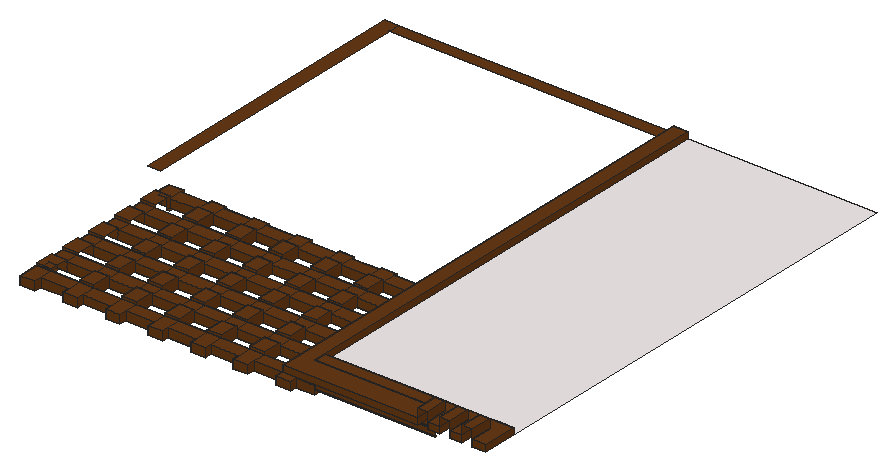
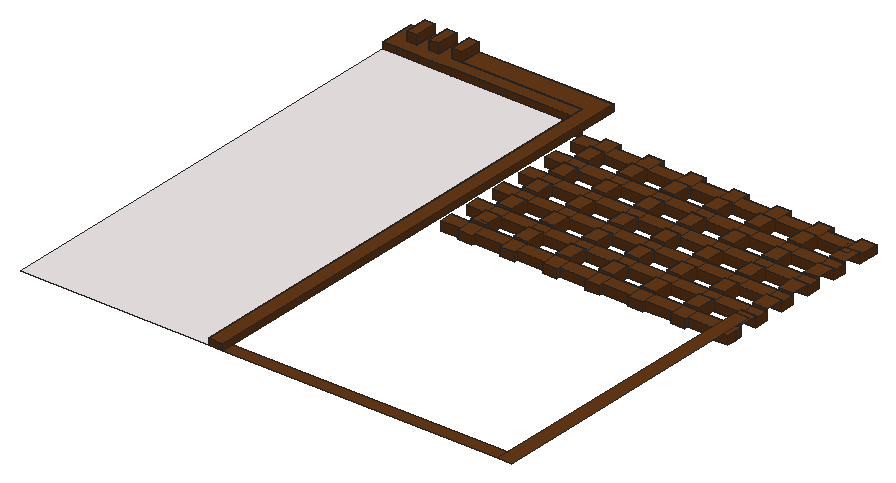
# SketchUp Ruby script. Lengths in inches.
U = 1.inch
M = Sketchup.active_model
def pt(a) = Geom::Point3d.new(a.map { |v| v * U })
def face(e, loops, mat)
  f = e.add_face(loops[0].map { |a| pt(a) })
  loops[1..].each { |l| e.add_face(l.map { |a| pt(a) }).erase! }
  f.material = f.back_material = mat if mat
  f
end
# faces: each face lists its corners as indices into pts; further lists are holes
def faces(e, pts, list, mat = nil) = list.each { |f| face(e, (f[0].is_a?(Array) ? f : [f]).map { |l| l.map { |i| pts[i] } }, mat) }
# xy, xz, yz: faces in a plane at the given z, y or x. An outline is a flat list of corners, or four numbers for a rectangle; further outlines are holes
def ring(l) = l.size == 4 ? [[l[0], l[1]], [l[2], l[1]], [l[2], l[3]], [l[0], l[3]]] : l.each_slice(2).to_a
def flat(e, list, mat, &to3) = list.each { |f| face(e, (f[0].is_a?(Array) ? f : [f]).map { |l| ring(l).map { |u, v| to3.(u, v) } }, mat) }
def xy(e, z, list, mat = nil) = flat(e, list, mat) { |x, y| [x, y, z] }
def xz(e, y, list, mat = nil) = flat(e, list, mat) { |x, z| [x, y, z] }
def yz(e, x, list, mat = nil) = flat(e, list, mat) { |y, z| [x, y, z] }
def lines(e, pts, list) = list.each { |a, b| e.add_line(pt(pts[a]), pt(pts[b])) }
# prism: a flat outline (further loops are holes) pulled along v
def prism(e, loops, v, mat = nil)
  f = face(e, loops, mat); d = Geom::Vector3d.new(v.map { |x| x * U })
  f.pushpull(f.normal.samedirection?(d) ? d.length : -d.length)
end
def box(e, o, s, mat = nil) = prism(e, [[o, [o[0] + s[0], o[1], o[2]], [o[0] + s[0], o[1] + s[1], o[2]], [o[0], o[1] + s[1], o[2]]]], [0, 0, s[2]], mat)
def at(x, y, z, deg = 0) = Geom::Transformation.translation(pt([x, y, z])) * Geom::Transformation.rotation(ORIGIN, Z_AXIS, deg.degrees)
def axes(o, x, y, z) = Geom::Transformation.new([*x, 0, *y, 0, *z, 0, *pt(o).to_a, 1])
def part(name) = M.definitions.add(name)
# library, detail: a bought-in or finely detailed component or shape, given as its bounding box
def library(name, o, s) = part(name).tap { |d| box(d.entities, o, s) }
def detail(e, o, s) = box(e.add_group.entities, o, s)
def put(e, d, t, mat = nil) = e.add_instance(d, t).tap { |i| i.material = mat if mat }
def group(e, t, mat = nil) = e.add_group.tap { |g| g.transformation = t; g.material = mat if mat }.entities
root = M.entities
M.materials.add("Generic").color = [102, 57, 22]
M.materials.add("Generic\#3").color = [243, 235, 235]
xy(root,493.22,[[27.12,205.01,30.01,205.01,30.01,218.57,19.57,218.57,19.57,208.75,27.12,208.75]],"Generic")
xy(root,493.4375,[[13.1875,47.8125,13.1875,67.5625,288.56,67.5625,288.56,54.375,270.5,54.375,270.5,47.8125,256.5625,47.8125,256.5625,54.375,229.93,54.375,229.93,47.8125,216,47.8125,216,54.375,189.37,54.375,189.37,47.8125,175.4375,47.8125,175.4375,54.375,148.81,54.375,148.81,47.8125,134.875,47.8125,134.875,54.375,108.25,54.375,108.25,47.8125,94.3125,47.8125,94.3125,54.375,67.68,54.375,67.68,47.8125,53.75,47.8125,53.75,54.375,27.12,54.375,27.12,47.8125],[53.75,67.5625,67.68,85.25],[94.3125,67.5625,108.25,85.25],[134.875,67.5625,148.81,85.25],[175.4375,67.5625,189.37,85.25],
  [216,67.5625,229.93,85.25],[256.5625,67.5625,270.5,85.25],[13.1875,85.25,288.56,98.4375],[53.75,98.4375,67.68,116.125],[94.3125,98.4375,108.25,116.125],
  [134.875,98.4375,148.81,116.125],[175.4375,98.4375,189.37,116.125],[216,98.4375,229.93,116.125],[256.5625,98.4375,270.5,116.125],[13.1875,116.125,288.56,129.3125],
  [53.75,129.3125,67.68,147],[94.3125,129.3125,108.25,147],[134.875,129.3125,148.81,147],[175.4375,129.3125,189.37,147],[216,129.3125,229.93,147],
  [256.5625,129.3125,270.5,147],[13.1875,147,288.56,160.1875],[53.75,160.1875,67.68,177.875],[94.3125,160.1875,108.25,177.875],[134.875,160.1875,148.81,177.875],
  [175.4375,160.1875,189.37,177.875],[216,160.1875,229.93,177.875],[256.5625,160.1875,270.5,177.875],[13.1875,177.875,288.56,191.0625],[53.75,191.0625,67.68,208.75],
  [94.3125,191.0625,108.25,208.75],[134.875,191.0625,148.81,208.75],[175.4375,191.0625,189.37,208.75],[216,191.0625,229.93,208.75],[256.5625,191.0625,270.5,208.75],
  [13.1875,208.75,13.1875,224.75,27.12,224.75,27.12,221.9375,53.75,221.9375,53.75,224.75,67.68,224.75,67.68,221.9375,94.3125,221.9375,94.3125,224.75,108.25,224.75,108.25,221.9375,134.875,221.9375,134.875,224.75,148.81,224.75,148.81,221.9375,175.4375,221.9375,175.4375,224.75,189.37,224.75,189.37,221.9375,216,221.9375,216,224.75,229.93,224.75,229.93,221.9375,256.5625,221.9375,256.5625,224.75,270.5,224.75,270.5,221.9375,288.56,221.9375,288.56,208.75]],"Generic")
xy(root,494.78,[[253.89,205.01,256.5625,205.01,256.5625,208.75,264.32,208.75,264.32,218.57,253.89,218.57]],"Generic")
xy(root,498,[[288.56,54.375,403,54.68]],"Generic")
xy(root,499,[[288.56,54.375,403,54.68]],"Generic")
xy(root,501.48,[[19.57,60.38,30.01,60.38,30.01,73.95,27.12,73.95,27.12,67.5625,19.57,67.5625]],"Generic")
xy(root,501.6,[[13.1875,47.8125,27.12,67.5625],[53.75,47.8125,67.68,67.5625],[94.3125,47.8125,108.25,67.5625],[134.875,47.8125,148.81,67.5625],[175.4375,47.8125,189.37,67.5625],
  [216,47.8125,229.93,67.5625],[256.5625,47.8125,270.5,67.5625],[27.12,54.375,53.75,67.5625],[67.68,54.375,94.3125,67.5625],[108.25,54.375,134.875,67.5625],
  [148.81,54.375,175.4375,67.5625],[189.37,54.375,216,67.5625],[229.93,54.375,256.5625,67.5625],[270.5,54.375,288.56,67.5625],[13.1875,85.25,27.12,98.4375],
  [27.12,85.25,53.75,98.4375],[53.75,85.25,67.68,98.4375],[67.68,85.25,94.3125,98.4375],[94.3125,85.25,108.25,98.4375],[108.25,85.25,134.875,98.4375],
  [134.875,85.25,148.81,98.4375],[148.81,85.25,175.4375,98.4375],[175.4375,85.25,189.37,98.4375],[189.37,85.25,216,98.4375],[216,85.25,229.93,98.4375],
  [229.93,85.25,256.5625,98.4375],[256.5625,85.25,270.5,98.4375],[270.5,85.25,288.56,98.4375],[13.1875,116.125,27.12,129.3125],[27.12,116.125,53.75,129.3125],
  [53.75,116.125,67.68,129.3125],[67.68,116.125,94.3125,129.3125],[94.3125,116.125,108.25,129.3125],[108.25,116.125,134.875,129.3125],[134.875,116.125,148.81,129.3125],
  [148.81,116.125,175.4375,129.3125],[175.4375,116.125,189.37,129.3125],[189.37,116.125,216,129.3125],[216,116.125,229.93,129.3125],[229.93,116.125,256.5625,129.3125],
  [256.5625,116.125,270.5,129.3125],[270.5,116.125,288.56,129.3125],[13.1875,147,27.12,160.1875],[27.12,147,53.75,160.1875],[53.75,147,67.68,160.1875],
  [67.68,147,94.3125,160.1875],[94.3125,147,108.25,160.1875],[108.25,147,134.875,160.1875],[134.875,147,148.81,160.1875],[148.81,147,175.4375,160.1875],
  [175.4375,147,189.37,160.1875],[189.37,147,216,160.1875],[216,147,229.93,160.1875],[229.93,147,256.5625,160.1875],[256.5625,147,270.5,160.1875],
  [270.5,147,288.56,160.1875],[13.1875,177.875,27.12,191.0625],[27.12,177.875,53.75,191.0625],[53.75,177.875,67.68,191.0625],[67.68,177.875,94.3125,191.0625],
  [94.3125,177.875,108.25,191.0625],[108.25,177.875,134.875,191.0625],[134.875,177.875,148.81,191.0625],[148.81,177.875,175.4375,191.0625],[175.4375,177.875,189.37,191.0625],
  [189.37,177.875,216,191.0625],[216,177.875,229.93,191.0625],[229.93,177.875,256.5625,191.0625],[256.5625,177.875,270.5,191.0625],[270.5,177.875,288.56,191.0625],
  [13.1875,208.75,27.12,224.75],[27.12,208.75,53.75,221.9375],[53.75,208.75,67.68,224.75],[67.68,208.75,94.3125,221.9375],[94.3125,208.75,108.25,224.75],
  [108.25,208.75,134.875,221.9375],[134.875,208.75,148.81,224.75],[148.81,208.75,175.4375,221.9375],[175.4375,208.75,189.37,224.75],[189.37,208.75,216,221.9375],
  [216,208.75,229.93,224.75],[229.93,208.75,256.5625,221.9375],[256.5625,208.75,270.5,224.75],[270.5,208.75,288.56,221.9375]],"Generic")
xy(root,503.72,[[13.1875,67.5625,19.57,67.5625,19.57,73.95,27.12,73.95,27.12,85.25,13.1875,85.25],[19.57,67.5625,27.12,73.95],[53.75,67.5625,67.68,85.25],[94.3125,67.5625,108.25,85.25],[134.875,67.5625,148.81,85.25],
  [175.4375,67.5625,189.37,85.25],[216,67.5625,229.93,85.25],[256.5625,67.5625,270.5,85.25],[13.1875,98.4375,27.12,116.125],[53.75,98.4375,67.68,116.125],
  [94.3125,98.4375,108.25,116.125],[134.875,98.4375,148.81,116.125],[175.4375,98.4375,189.37,116.125],[216,98.4375,229.93,116.125],[256.5625,98.4375,270.5,116.125],
  [13.1875,129.3125,27.12,147],[53.75,129.3125,67.68,147],[94.3125,129.3125,108.25,147],[134.875,129.3125,148.81,147],[175.4375,129.3125,189.37,147],
  [216,129.3125,229.93,147],[256.5625,129.3125,270.5,147],[13.1875,160.1875,27.12,177.875],[53.75,160.1875,67.68,177.875],[94.3125,160.1875,108.25,177.875],
  [134.875,160.1875,148.81,177.875],[175.4375,160.1875,189.37,177.875],[216,160.1875,229.93,177.875],[256.5625,160.1875,270.5,177.875],[13.1875,191.0625,27.12,191.0625,27.12,205.01,19.57,205.01,19.57,208.75,13.1875,208.75],
  [53.75,191.0625,67.68,208.75],[94.3125,191.0625,108.25,208.75],[134.875,191.0625,148.81,208.75],[175.4375,191.0625,189.37,208.75],[216,191.0625,229.93,208.75],
  [256.5625,191.0625,270.5,191.0625,270.5,208.75,264.32,208.75,264.32,205.01,256.5625,205.01],[19.57,205.01,27.12,208.75],[256.5625,205.01,264.32,208.75]],"Generic")
xy(root,504.3125,[[288.56,54.375,403,54.68]],"Generic")
xy(root,505.3125,[[288.56,54.375,403,54.68]],"Generic")
xy(root,510.625,[[288.56,54.375,403,54.68]],"Generic")
xy(root,511.625,[[288.56,54.375,403,54.68]],"Generic")
xy(root,517.125,[[274.62,33.625,274.62,486.875,288.56,486.875,288.56,54.375,403,54.375,403,33.625],[412.5,33.625,424.1875,54.375],[433.6875,33.625,445.375,54.375],[454.875,33.625,467.875,54.375],[288.56,54.375,467.875,66.4375],
  [0,215.5,13.1875,498.375],[13.1875,486.875,274.62,498.375],[274.62,486.875,288.56,498.375]],"Generic")
xy(root,517.125,[[288.56,66.4375,467.875,498.375]],"Generic\#3")
xy(root,523.25,[[274.62,33.625,403,33.625,403,54.375,288.56,54.375,288.56,498.375,274.62,498.375],[412.5,33.625,424.1875,33.625,424.1875,54.375,433.6875,54.375,433.6875,33.625,445.375,33.625,445.375,54.375,454.875,54.375,454.875,33.625,467.875,33.625,467.875,66.4375,288.56,66.4375,288.56,54.375,412.5,54.375]],"Generic")
xy(root,531.8125,[[403,33.625,412.5,54.375],[424.1875,33.625,433.6875,54.375],[445.375,33.625,454.875,54.375]],"Generic")
xz(root,33.625,[[274.62,517.125,403,523.25],[412.5,517.125,424.1875,523.25],[433.6875,517.125,445.375,523.25],[454.875,517.125,467.875,523.25]],"Generic")
xz(root,47.8125,[[13.1875,493.4375,27.12,501.6],[53.75,493.4375,67.68,501.6],[94.3125,493.4375,108.25,501.6],[134.875,493.4375,148.81,501.6],[175.4375,493.4375,189.37,501.6],
  [216,493.4375,229.93,501.6],[256.5625,493.4375,270.5,501.6]],"Generic")
xz(root,54.375,[[27.12,493.4375,53.75,501.6],[67.68,493.4375,94.3125,501.6],[108.25,493.4375,134.875,501.6],[148.81,493.4375,175.4375,501.6],[189.37,493.4375,216,501.6],
  [229.93,493.4375,256.5625,501.6],[270.5,493.4375,288.56,501.6],[288.56,499,403,504.3125],[288.56,505.3125,403,510.625],[288.56,511.625,403,517.125],
  [288.56,517.125,403,523.25],[403,517.125,412.5,523.25],[424.1875,517.125,433.6875,523.25],[445.375,517.125,454.875,523.25],[403,523.25,412.5,531.8125],
  [424.1875,523.25,433.6875,531.8125],[445.375,523.25,454.875,531.8125]],"Generic")
xz(root,54.68,[[288.56,498,403,499],[288.56,504.3125,403,505.3125],[288.56,510.625,403,511.625]],"Generic")
xz(root,66.4375,[[288.56,517.125,403,523.25],[403,517.125,412.5,523.25],[412.5,517.125,424.1875,523.25],[424.1875,517.125,433.6875,523.25],[433.6875,517.125,445.375,523.25],
  [445.375,517.125,454.875,523.25],[454.875,517.125,467.875,523.25]],"Generic")
xz(root,67.5625,[[13.1875,493.4375,13.1875,501.6,19.57,501.6,19.57,501.48,27.12,501.48,27.12,493.4375],[27.12,493.4375,53.75,501.6],[53.75,493.4375,67.68,501.6],[67.68,493.4375,94.3125,501.6],[94.3125,493.4375,108.25,501.6],
  [108.25,493.4375,134.875,501.6],[134.875,493.4375,148.81,501.6],[148.81,493.4375,175.4375,501.6],[175.4375,493.4375,189.37,501.6],[189.37,493.4375,216,501.6],
  [216,493.4375,229.93,501.6],[229.93,493.4375,256.5625,501.6],[256.5625,493.4375,270.5,501.6],[270.5,493.4375,288.56,501.6],[19.57,501.48,27.12,501.6],
  [13.1875,501.6,19.57,503.72],[19.57,501.6,27.12,503.72],[53.75,501.6,67.68,503.72],[94.3125,501.6,108.25,503.72],[134.875,501.6,148.81,503.72],
  [175.4375,501.6,189.37,503.72],[216,501.6,229.93,503.72],[256.5625,501.6,270.5,503.72]],"Generic")
xz(root,85.25,[[13.1875,493.4375,27.12,501.6],[27.12,493.4375,53.75,501.6],[53.75,493.4375,67.68,501.6],[67.68,493.4375,94.3125,501.6],[94.3125,493.4375,108.25,501.6],
  [108.25,493.4375,134.875,501.6],[134.875,493.4375,148.81,501.6],[148.81,493.4375,175.4375,501.6],[175.4375,493.4375,189.37,501.6],[189.37,493.4375,216,501.6],
  [216,493.4375,229.93,501.6],[229.93,493.4375,256.5625,501.6],[256.5625,493.4375,270.5,501.6],[270.5,493.4375,288.56,501.6],[13.1875,501.6,27.12,503.72],
  [53.75,501.6,67.68,503.72],[94.3125,501.6,108.25,503.72],[134.875,501.6,148.81,503.72],[175.4375,501.6,189.37,503.72],[216,501.6,229.93,503.72],
  [256.5625,501.6,270.5,503.72]],"Generic")
xz(root,98.4375,[[13.1875,493.4375,27.12,501.6],[27.12,493.4375,53.75,501.6],[53.75,493.4375,67.68,501.6],[67.68,493.4375,94.3125,501.6],[94.3125,493.4375,108.25,501.6],
  [108.25,493.4375,134.875,501.6],[134.875,493.4375,148.81,501.6],[148.81,493.4375,175.4375,501.6],[175.4375,493.4375,189.37,501.6],[189.37,493.4375,216,501.6],
  [216,493.4375,229.93,501.6],[229.93,493.4375,256.5625,501.6],[256.5625,493.4375,270.5,501.6],[270.5,493.4375,288.56,501.6],[13.1875,501.6,27.12,503.72],
  [53.75,501.6,67.68,503.72],[94.3125,501.6,108.25,503.72],[134.875,501.6,148.81,503.72],[175.4375,501.6,189.37,503.72],[216,501.6,229.93,503.72],
  [256.5625,501.6,270.5,503.72]],"Generic")
xz(root,116.125,[[13.1875,493.4375,27.12,501.6],[27.12,493.4375,53.75,501.6],[53.75,493.4375,67.68,501.6],[67.68,493.4375,94.3125,501.6],[94.3125,493.4375,108.25,501.6],
  [108.25,493.4375,134.875,501.6],[134.875,493.4375,148.81,501.6],[148.81,493.4375,175.4375,501.6],[175.4375,493.4375,189.37,501.6],[189.37,493.4375,216,501.6],
  [216,493.4375,229.93,501.6],[229.93,493.4375,256.5625,501.6],[256.5625,493.4375,270.5,501.6],[270.5,493.4375,288.56,501.6],[13.1875,501.6,27.12,503.72],
  [53.75,501.6,67.68,503.72],[94.3125,501.6,108.25,503.72],[134.875,501.6,148.81,503.72],[175.4375,501.6,189.37,503.72],[216,501.6,229.93,503.72],
  [256.5625,501.6,270.5,503.72]],"Generic")
xz(root,129.3125,[[13.1875,493.4375,27.12,501.6],[27.12,493.4375,53.75,501.6],[53.75,493.4375,67.68,501.6],[67.68,493.4375,94.3125,501.6],[94.3125,493.4375,108.25,501.6],
  [108.25,493.4375,134.875,501.6],[134.875,493.4375,148.81,501.6],[148.81,493.4375,175.4375,501.6],[175.4375,493.4375,189.37,501.6],[189.37,493.4375,216,501.6],
  [216,493.4375,229.93,501.6],[229.93,493.4375,256.5625,501.6],[256.5625,493.4375,270.5,501.6],[270.5,493.4375,288.56,501.6],[13.1875,501.6,27.12,503.72],
  [53.75,501.6,67.68,503.72],[94.3125,501.6,108.25,503.72],[134.875,501.6,148.81,503.72],[175.4375,501.6,189.37,503.72],[216,501.6,229.93,503.72],
  [256.5625,501.6,270.5,503.72]],"Generic")
xz(root,147,[[13.1875,493.4375,27.12,501.6],[27.12,493.4375,53.75,501.6],[53.75,493.4375,67.68,501.6],[67.68,493.4375,94.3125,501.6],[94.3125,493.4375,108.25,501.6],
  [108.25,493.4375,134.875,501.6],[134.875,493.4375,148.81,501.6],[148.81,493.4375,175.4375,501.6],[175.4375,493.4375,189.37,501.6],[189.37,493.4375,216,501.6],
  [216,493.4375,229.93,501.6],[229.93,493.4375,256.5625,501.6],[256.5625,493.4375,270.5,501.6],[270.5,493.4375,288.56,501.6],[13.1875,501.6,27.12,503.72],
  [53.75,501.6,67.68,503.72],[94.3125,501.6,108.25,503.72],[134.875,501.6,148.81,503.72],[175.4375,501.6,189.37,503.72],[216,501.6,229.93,503.72],
  [256.5625,501.6,270.5,503.72]],"Generic")
xz(root,160.1875,[[13.1875,493.4375,27.12,501.6],[27.12,493.4375,53.75,501.6],[53.75,493.4375,67.68,501.6],[67.68,493.4375,94.3125,501.6],[94.3125,493.4375,108.25,501.6],
  [108.25,493.4375,134.875,501.6],[134.875,493.4375,148.81,501.6],[148.81,493.4375,175.4375,501.6],[175.4375,493.4375,189.37,501.6],[189.37,493.4375,216,501.6],
  [216,493.4375,229.93,501.6],[229.93,493.4375,256.5625,501.6],[256.5625,493.4375,270.5,501.6],[270.5,493.4375,288.56,501.6],[13.1875,501.6,27.12,503.72],
  [53.75,501.6,67.68,503.72],[94.3125,501.6,108.25,503.72],[134.875,501.6,148.81,503.72],[175.4375,501.6,189.37,503.72],[216,501.6,229.93,503.72],
  [256.5625,501.6,270.5,503.72]],"Generic")
xz(root,177.875,[[13.1875,493.4375,27.12,501.6],[27.12,493.4375,53.75,501.6],[53.75,493.4375,67.68,501.6],[67.68,493.4375,94.3125,501.6],[94.3125,493.4375,108.25,501.6],
  [108.25,493.4375,134.875,501.6],[134.875,493.4375,148.81,501.6],[148.81,493.4375,175.4375,501.6],[175.4375,493.4375,189.37,501.6],[189.37,493.4375,216,501.6],
  [216,493.4375,229.93,501.6],[229.93,493.4375,256.5625,501.6],[256.5625,493.4375,270.5,501.6],[270.5,493.4375,288.56,501.6],[13.1875,501.6,27.12,503.72],
  [53.75,501.6,67.68,503.72],[94.3125,501.6,108.25,503.72],[134.875,501.6,148.81,503.72],[175.4375,501.6,189.37,503.72],[216,501.6,229.93,503.72],
  [256.5625,501.6,270.5,503.72]],"Generic")
xz(root,191.0625,[[13.1875,493.4375,27.12,501.6],[27.12,493.4375,53.75,501.6],[53.75,493.4375,67.68,501.6],[67.68,493.4375,94.3125,501.6],[94.3125,493.4375,108.25,501.6],
  [108.25,493.4375,134.875,501.6],[134.875,493.4375,148.81,501.6],[148.81,493.4375,175.4375,501.6],[175.4375,493.4375,189.37,501.6],[189.37,493.4375,216,501.6],
  [216,493.4375,229.93,501.6],[229.93,493.4375,256.5625,501.6],[256.5625,493.4375,270.5,501.6],[270.5,493.4375,288.56,501.6],[13.1875,501.6,27.12,503.72],
  [53.75,501.6,67.68,503.72],[94.3125,501.6,108.25,503.72],[134.875,501.6,148.81,503.72],[175.4375,501.6,189.37,503.72],[216,501.6,229.93,503.72],
  [256.5625,501.6,270.5,503.72]],"Generic")
xz(root,208.75,[[19.57,493.22,27.12,493.4375],[13.1875,493.4375,19.57,501.6],[19.57,493.4375,27.12,501.6],[27.12,493.4375,53.75,501.6],[53.75,493.4375,67.68,501.6],
  [67.68,493.4375,94.3125,501.6],[94.3125,493.4375,108.25,501.6],[108.25,493.4375,134.875,501.6],[134.875,493.4375,148.81,501.6],[148.81,493.4375,175.4375,501.6],
  [175.4375,493.4375,189.37,501.6],[189.37,493.4375,216,501.6],[216,493.4375,229.93,501.6],[229.93,493.4375,256.5625,501.6],[256.5625,493.4375,270.5,493.4375,270.5,501.6,264.32,501.6,264.32,494.78,256.5625,494.78],
  [270.5,493.4375,288.56,501.6],[256.5625,494.78,264.32,501.6],[13.1875,501.6,19.57,503.72],[19.57,501.6,27.12,503.72],[53.75,501.6,67.68,503.72],
  [94.3125,501.6,108.25,503.72],[134.875,501.6,148.81,503.72],[175.4375,501.6,189.37,503.72],[216,501.6,229.93,503.72],[256.5625,501.6,264.32,503.72],
  [264.32,501.6,270.5,503.72]],"Generic")
xz(root,221.9375,[[27.12,493.4375,53.75,501.6],[67.68,493.4375,94.3125,501.6],[108.25,493.4375,134.875,501.6],[148.81,493.4375,175.4375,501.6],[189.37,493.4375,216,501.6],
  [229.93,493.4375,256.5625,501.6],[270.5,493.4375,288.56,501.6]],"Generic")
xz(root,224.75,[[13.1875,493.4375,27.12,501.6],[53.75,493.4375,67.68,501.6],[94.3125,493.4375,108.25,501.6],[134.875,493.4375,148.81,501.6],[175.4375,493.4375,189.37,501.6],
  [216,493.4375,229.93,501.6],[256.5625,493.4375,270.5,501.6]],"Generic")
xz(root,498.375,[[274.62,517.125,288.56,523.25]],"Generic")
yz(root,13.1875,[[47.8125,493.4375,67.5625,501.6],[85.25,493.4375,98.4375,501.6],[116.125,493.4375,129.3125,501.6],[147,493.4375,160.1875,501.6],[177.875,493.4375,191.0625,501.6],
  [208.75,493.4375,215.5,501.6],[215.5,493.4375,224.75,501.6]],"Generic")
yz(root,27.12,[[205.01,493.22,208.75,503.72],[47.8125,493.4375,54.375,501.6],[221.9375,493.4375,224.75,501.6],[67.5625,501.48,73.95,503.72]],"Generic")
yz(root,53.75,[[47.8125,493.4375,54.375,501.6],[67.5625,493.4375,85.25,503.72],[98.4375,493.4375,116.125,503.72],[129.3125,493.4375,147,503.72],[160.1875,493.4375,177.875,503.72],
  [191.0625,493.4375,208.75,503.72],[221.9375,493.4375,224.75,501.6]],"Generic")
yz(root,67.68,[[47.8125,493.4375,54.375,501.6],[67.5625,493.4375,85.25,503.72],[98.4375,493.4375,116.125,503.72],[129.3125,493.4375,147,503.72],[160.1875,493.4375,177.875,503.72],
  [191.0625,493.4375,208.75,503.72],[221.9375,493.4375,224.75,501.6]],"Generic")
yz(root,94.3125,[[47.8125,493.4375,54.375,501.6],[67.5625,493.4375,85.25,503.72],[98.4375,493.4375,116.125,503.72],[129.3125,493.4375,147,503.72],[160.1875,493.4375,177.875,503.72],
  [191.0625,493.4375,208.75,503.72],[221.9375,493.4375,224.75,501.6]],"Generic")
yz(root,108.25,[[47.8125,493.4375,54.375,501.6],[67.5625,493.4375,85.25,503.72],[98.4375,493.4375,116.125,503.72],[129.3125,493.4375,147,503.72],[160.1875,493.4375,177.875,503.72],
  [191.0625,493.4375,208.75,503.72],[221.9375,493.4375,224.75,501.6]],"Generic")
yz(root,134.875,[[47.8125,493.4375,54.375,501.6],[67.5625,493.4375,85.25,503.72],[98.4375,493.4375,116.125,503.72],[129.3125,493.4375,147,503.72],[160.1875,493.4375,177.875,503.72],
  [191.0625,493.4375,208.75,503.72],[221.9375,493.4375,224.75,501.6]],"Generic")
yz(root,148.81,[[47.8125,493.4375,54.375,501.6],[67.5625,493.4375,85.25,503.72],[98.4375,493.4375,116.125,503.72],[129.3125,493.4375,147,503.72],[160.1875,493.4375,177.875,503.72],
  [191.0625,493.4375,208.75,503.72],[221.9375,493.4375,224.75,501.6]],"Generic")
yz(root,175.4375,[[47.8125,493.4375,54.375,501.6],[67.5625,493.4375,85.25,503.72],[98.4375,493.4375,116.125,503.72],[129.3125,493.4375,147,503.72],[160.1875,493.4375,177.875,503.72],
  [191.0625,493.4375,208.75,503.72],[221.9375,493.4375,224.75,501.6]],"Generic")
yz(root,189.37,[[47.8125,493.4375,54.375,501.6],[67.5625,493.4375,85.25,503.72],[98.4375,493.4375,116.125,503.72],[129.3125,493.4375,147,503.72],[160.1875,493.4375,177.875,503.72],
  [191.0625,493.4375,208.75,503.72],[221.9375,493.4375,224.75,501.6]],"Generic")
yz(root,216,[[47.8125,493.4375,54.375,501.6],[67.5625,493.4375,85.25,503.72],[98.4375,493.4375,116.125,503.72],[129.3125,493.4375,147,503.72],[160.1875,493.4375,177.875,503.72],
  [191.0625,493.4375,208.75,503.72],[221.9375,493.4375,224.75,501.6]],"Generic")
yz(root,229.93,[[47.8125,493.4375,54.375,501.6],[67.5625,493.4375,85.25,503.72],[98.4375,493.4375,116.125,503.72],[129.3125,493.4375,147,503.72],[160.1875,493.4375,177.875,503.72],
  [191.0625,493.4375,208.75,503.72],[221.9375,493.4375,224.75,501.6]],"Generic")
yz(root,256.5625,[[47.8125,493.4375,54.375,501.6],[67.5625,493.4375,85.25,503.72],[98.4375,493.4375,116.125,503.72],[129.3125,493.4375,147,503.72],[160.1875,493.4375,177.875,503.72],
  [191.0625,493.4375,191.0625,503.72,205.01,503.72,205.01,494.78,208.75,494.78,208.75,493.4375],[221.9375,493.4375,224.75,501.6],[205.01,494.78,208.75,503.72]],"Generic")
yz(root,270.5,[[47.8125,493.4375,54.375,501.6],[67.5625,493.4375,85.25,503.72],[98.4375,493.4375,116.125,503.72],[129.3125,493.4375,147,503.72],[160.1875,493.4375,177.875,503.72],
  [191.0625,493.4375,208.75,503.72],[221.9375,493.4375,224.75,501.6]],"Generic")
yz(root,274.62,[[33.625,517.125,498.375,523.25]],"Generic")
yz(root,288.56,[[54.375,493.4375,54.375,498,54.68,498,54.68,499,54.375,499,54.375,501.6,67.5625,501.6,67.5625,493.4375],[54.375,498,54.68,499],[54.375,517.125,66.4375,523.25],[66.4375,517.125,498.375,523.25]],"Generic")
yz(root,403,[[54.375,498,54.68,499],[54.375,504.3125,54.68,505.3125],[54.375,510.625,54.68,511.625],[33.625,517.125,54.375,523.25],[33.625,523.25,54.375,531.8125]],"Generic")
yz(root,412.5,[[33.625,517.125,54.375,523.25],[33.625,523.25,54.375,531.8125]],"Generic")
yz(root,424.1875,[[33.625,517.125,54.375,523.25],[33.625,523.25,54.375,531.8125]],"Generic")
yz(root,433.6875,[[33.625,517.125,54.375,523.25],[33.625,523.25,54.375,531.8125]],"Generic")
yz(root,445.375,[[33.625,517.125,54.375,523.25],[33.625,523.25,54.375,531.8125]],"Generic")
yz(root,454.875,[[33.625,517.125,54.375,523.25],[33.625,523.25,54.375,531.8125]],"Generic")
yz(root,467.875,[[33.625,517.125,66.4375,523.25]],"Generic")
